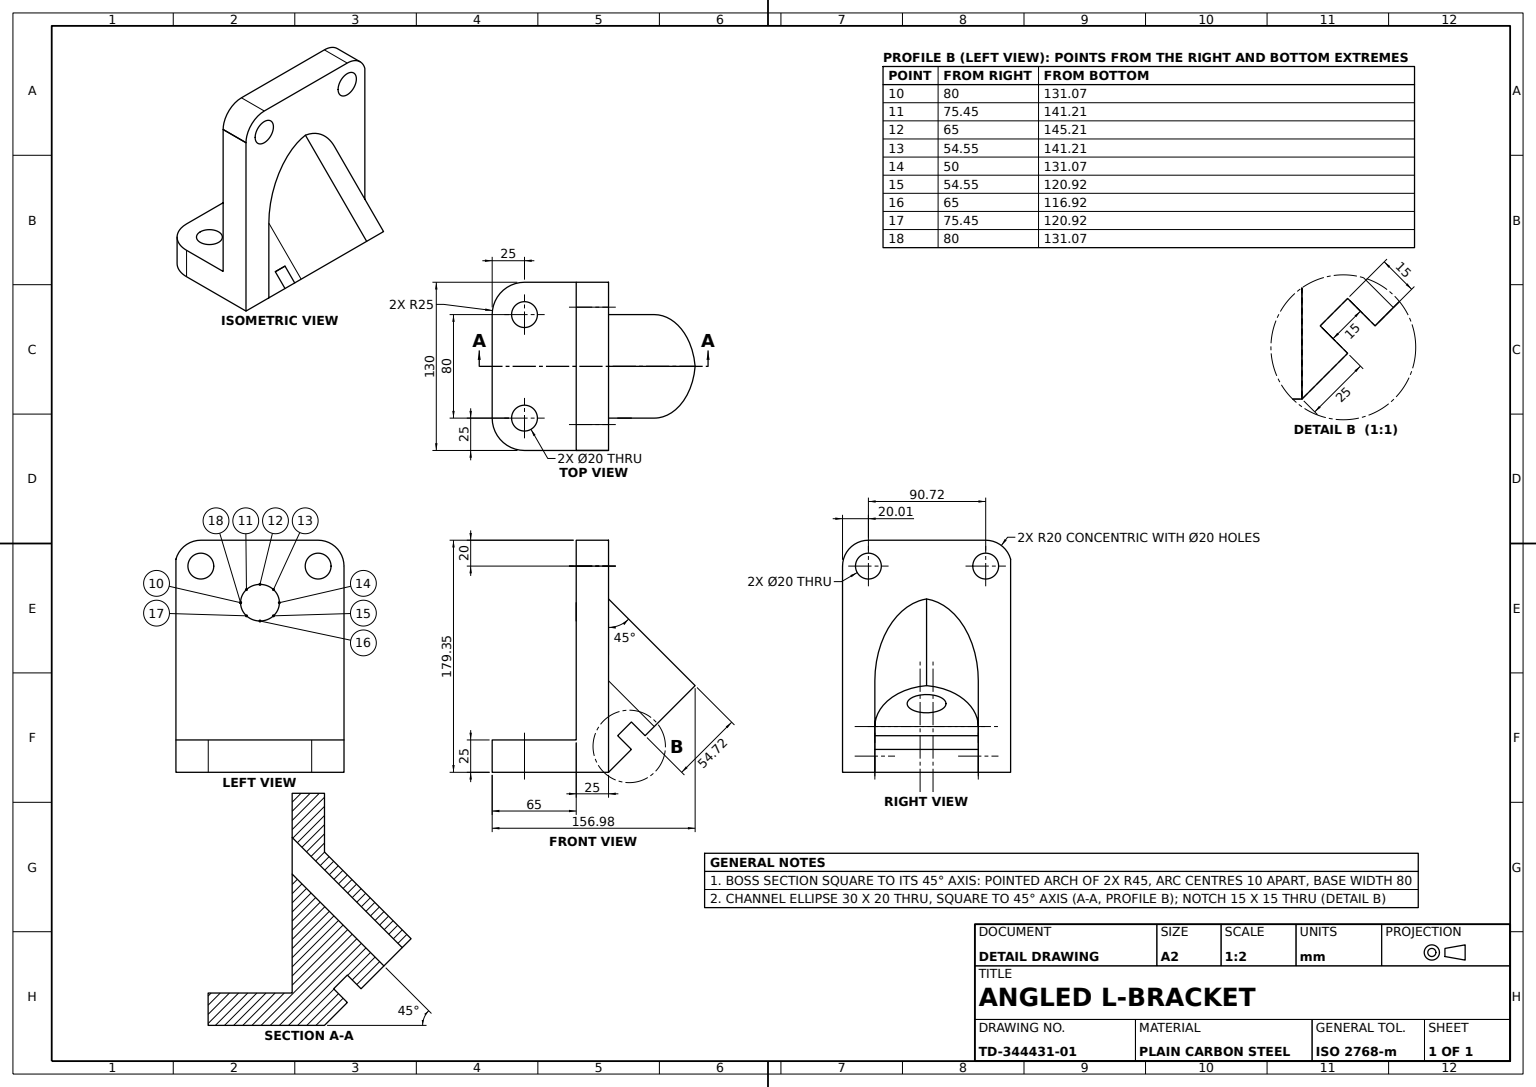
ISO-10303-21;
HEADER;
FILE_DESCRIPTION((''),'2;1');
FILE_NAME('','',(''),(''),'','','');
FILE_SCHEMA(('AUTOMOTIVE_DESIGN'));
ENDSEC;
DATA;
#1=APPLICATION_CONTEXT('');
#2=PRODUCT_CONTEXT('',#1,'mechanical');
#3=PRODUCT('','','',(#2));
#4=PRODUCT_DEFINITION_FORMATION('','',#3);
#5=PRODUCT_DEFINITION_CONTEXT('',#1,'design');
#6=PRODUCT_DEFINITION('','',#4,#5);
#7=PRODUCT_DEFINITION_SHAPE('','',#6);
#8=(LENGTH_UNIT()NAMED_UNIT(*)SI_UNIT(.MILLI.,.METRE.));
#9=(NAMED_UNIT(*)PLANE_ANGLE_UNIT()SI_UNIT($,.RADIAN.));
#10=(NAMED_UNIT(*)SI_UNIT($,.STERADIAN.)SOLID_ANGLE_UNIT());
#11=UNCERTAINTY_MEASURE_WITH_UNIT(LENGTH_MEASURE(1.E-05),#8,'distance_accuracy_value','');
#12=(GEOMETRIC_REPRESENTATION_CONTEXT(3)GLOBAL_UNCERTAINTY_ASSIGNED_CONTEXT((#11))GLOBAL_UNIT_ASSIGNED_CONTEXT((#8,#9,#10))REPRESENTATION_CONTEXT('',''));
#13=CARTESIAN_POINT('',(60.702747,0.,-23.512021));
#14=VERTEX_POINT('',#13);
#15=CARTESIAN_POINT('',(60.702747,25.,-23.512021));
#16=VERTEX_POINT('',#15);
#17=CARTESIAN_POINT('',(60.702747,-51.,-23.512021));
#18=DIRECTION('',(0.,1.,0.));
#19=VECTOR('',#18,1000.);
#20=LINE('',#17,#19);
#21=EDGE_CURVE('',#14,#16,#20,.T.);
#22=ORIENTED_EDGE('',*,*,#21,.F.);
#23=CARTESIAN_POINT('',(60.702747,0.,-43.512021));
#24=VERTEX_POINT('',#23);
#25=CARTESIAN_POINT('',(60.702747,0.,-33.512021));
#26=DIRECTION('',(0.,-1.,0.));
#27=DIRECTION('',(0.,0.,1.));
#28=AXIS2_PLACEMENT_3D('',#25,#26,#27);
#29=CIRCLE('',#28,10.);
#30=EDGE_CURVE('',#14,#24,#29,.T.);
#31=ORIENTED_EDGE('',*,*,#30,.T.);
#32=CARTESIAN_POINT('',(60.702747,25.,-43.512021));
#33=VERTEX_POINT('',#32);
#34=CARTESIAN_POINT('',(60.702747,-51.,-43.512021));
#35=LINE('',#34,#19);
#36=EDGE_CURVE('',#24,#33,#35,.T.);
#37=ORIENTED_EDGE('',*,*,#36,.T.);
#38=CARTESIAN_POINT('',(60.702747,25.,-33.512021));
#39=AXIS2_PLACEMENT_3D('',#38,#26,#27);
#40=CIRCLE('',#39,10.);
#41=EDGE_CURVE('',#16,#33,#40,.T.);
#42=ORIENTED_EDGE('',*,*,#41,.F.);
#43=EDGE_LOOP('',(#22,#31,#37,#42));
#44=FACE_OUTER_BOUND('',#43,.T.);
#45=CARTESIAN_POINT('',(60.702747,-51.,-33.512021));
#46=AXIS2_PLACEMENT_3D('',#45,#18,#27);
#47=CYLINDRICAL_SURFACE('',#46,10.);
#48=ADVANCED_FACE('',(#44),#47,.F.);
#49=CARTESIAN_POINT('',(85.702747,159.350288,-98.512021));
#50=VERTEX_POINT('',#49);
#51=CARTESIAN_POINT('',(85.702747,0.,-98.512021));
#52=VERTEX_POINT('',#51);
#53=CARTESIAN_POINT('',(85.702747,25.,-98.512021));
#54=VECTOR('',#26,1000.);
#55=LINE('',#53,#54);
#56=EDGE_CURVE('',#50,#52,#55,.T.);
#57=ORIENTED_EDGE('',*,*,#56,.F.);
#58=CARTESIAN_POINT('',(85.702747,159.350288,-73.512021));
#59=VERTEX_POINT('',#58);
#60=CARTESIAN_POINT('',(85.702747,159.350288,77.487979));
#61=DIRECTION('',(0.,0.,-1.));
#62=VECTOR('',#61,1000.);
#63=LINE('',#60,#62);
#64=EDGE_CURVE('',#59,#50,#63,.T.);
#65=ORIENTED_EDGE('',*,*,#64,.F.);
#66=CARTESIAN_POINT('',(85.702747,25.,-73.512021));
#67=VERTEX_POINT('',#66);
#68=CARTESIAN_POINT('',(85.702747,329.,-73.512021));
#69=LINE('',#68,#54);
#70=EDGE_CURVE('',#59,#67,#69,.T.);
#71=ORIENTED_EDGE('',*,*,#70,.T.);
#72=CARTESIAN_POINT('',(85.702747,25.,-33.512021));
#73=VERTEX_POINT('',#72);
#74=LINE('',#72,#62);
#75=EDGE_CURVE('',#73,#67,#74,.T.);
#76=ORIENTED_EDGE('',*,*,#75,.F.);
#77=CARTESIAN_POINT('',(85.702747,0.,-33.512021));
#78=VERTEX_POINT('',#77);
#79=LINE('',#72,#54);
#80=EDGE_CURVE('',#73,#78,#79,.T.);
#81=ORIENTED_EDGE('',*,*,#80,.T.);
#82=LINE('',#77,#62);
#83=EDGE_CURVE('',#78,#52,#82,.T.);
#84=ORIENTED_EDGE('',*,*,#83,.T.);
#85=EDGE_LOOP('',(#57,#65,#71,#76,#81,#84));
#86=FACE_OUTER_BOUND('',#85,.T.);
#87=DIRECTION('',(-1.,0.,0.));
#88=AXIS2_PLACEMENT_3D('',#72,#87,#27);
#89=PLANE('',#88);
#90=ADVANCED_FACE('',(#86),#89,.F.);
#91=CARTESIAN_POINT('',(-44.297253,164.722344,-98.512021));
#92=VERTEX_POINT('',#91);
#93=CARTESIAN_POINT('',(-44.297253,164.722344,-73.512021));
#94=VERTEX_POINT('',#93);
#95=CARTESIAN_POINT('',(-44.297253,164.722344,77.487979));
#96=VECTOR('',#27,1000.);
#97=LINE('',#95,#96);
#98=EDGE_CURVE('',#92,#94,#97,.T.);
#99=ORIENTED_EDGE('',*,*,#98,.T.);
#100=CARTESIAN_POINT('',(-25.032232,179.350288,-73.512021));
#101=VERTEX_POINT('',#100);
#102=CARTESIAN_POINT('',(-25.032232,159.350288,-73.512021));
#103=AXIS2_PLACEMENT_3D('',#102,#61,#87);
#104=CIRCLE('',#103,20.);
#105=EDGE_CURVE('',#94,#101,#104,.T.);
#106=ORIENTED_EDGE('',*,*,#105,.T.);
#107=CARTESIAN_POINT('',(-25.032232,179.350288,-98.512021));
#108=VERTEX_POINT('',#107);
#109=CARTESIAN_POINT('',(-25.032232,179.350288,77.487979));
#110=LINE('',#109,#62);
#111=EDGE_CURVE('',#101,#108,#110,.T.);
#112=ORIENTED_EDGE('',*,*,#111,.T.);
#113=CARTESIAN_POINT('',(-25.032232,159.350288,-98.512021));
#114=AXIS2_PLACEMENT_3D('',#113,#61,#87);
#115=CIRCLE('',#114,20.);
#116=EDGE_CURVE('',#92,#108,#115,.T.);
#117=ORIENTED_EDGE('',*,*,#116,.F.);
#118=EDGE_LOOP('',(#99,#106,#112,#117));
#119=FACE_OUTER_BOUND('',#118,.T.);
#120=CARTESIAN_POINT('',(-25.032232,159.350288,77.487979));
#121=AXIS2_PLACEMENT_3D('',#120,#61,#87);
#122=CYLINDRICAL_SURFACE('',#121,20.);
#123=ADVANCED_FACE('',(#119),#122,.T.);
#124=CARTESIAN_POINT('',(60.702747,25.,-8.512021));
#125=VERTEX_POINT('',#124);
#126=CARTESIAN_POINT('',(60.702747,0.,-8.512021));
#127=VERTEX_POINT('',#126);
#128=LINE('',#124,#54);
#129=EDGE_CURVE('',#125,#127,#128,.T.);
#130=ORIENTED_EDGE('',*,*,#129,.F.);
#131=CARTESIAN_POINT('',(-19.297253,25.,-8.512021));
#132=VERTEX_POINT('',#131);
#133=DIRECTION('',(1.,0.,0.));
#134=VECTOR('',#133,1000.);
#135=LINE('',#131,#134);
#136=EDGE_CURVE('',#132,#125,#135,.T.);
#137=ORIENTED_EDGE('',*,*,#136,.F.);
#138=CARTESIAN_POINT('',(-19.297253,0.,-8.512021));
#139=VERTEX_POINT('',#138);
#140=LINE('',#131,#54);
#141=EDGE_CURVE('',#132,#139,#140,.T.);
#142=ORIENTED_EDGE('',*,*,#141,.T.);
#143=LINE('',#138,#134);
#144=EDGE_CURVE('',#139,#127,#143,.T.);
#145=ORIENTED_EDGE('',*,*,#144,.T.);
#146=EDGE_LOOP('',(#130,#137,#142,#145));
#147=FACE_OUTER_BOUND('',#146,.T.);
#148=AXIS2_PLACEMENT_3D('',#131,#61,#87);
#149=PLANE('',#148);
#150=ADVANCED_FACE('',(#147),#149,.F.);
#151=ORIENTED_EDGE('',*,*,#141,.F.);
#152=CARTESIAN_POINT('',(-44.297253,25.,-33.512021));
#153=VERTEX_POINT('',#152);
#154=CARTESIAN_POINT('',(-19.297253,25.,-33.512021));
#155=AXIS2_PLACEMENT_3D('',#154,#18,#27);
#156=CIRCLE('',#155,25.);
#157=EDGE_CURVE('',#153,#132,#156,.T.);
#158=ORIENTED_EDGE('',*,*,#157,.F.);
#159=CARTESIAN_POINT('',(-44.297253,0.,-33.512021));
#160=VERTEX_POINT('',#159);
#161=LINE('',#152,#54);
#162=EDGE_CURVE('',#153,#160,#161,.T.);
#163=ORIENTED_EDGE('',*,*,#162,.T.);
#164=CARTESIAN_POINT('',(-19.297253,0.,-33.512021));
#165=AXIS2_PLACEMENT_3D('',#164,#18,#27);
#166=CIRCLE('',#165,25.);
#167=EDGE_CURVE('',#160,#139,#166,.T.);
#168=ORIENTED_EDGE('',*,*,#167,.T.);
#169=EDGE_LOOP('',(#151,#158,#163,#168));
#170=FACE_OUTER_BOUND('',#169,.T.);
#171=AXIS2_PLACEMENT_3D('',#154,#26,#61);
#172=CYLINDRICAL_SURFACE('',#171,25.);
#173=ADVANCED_FACE('',(#170),#172,.T.);
#174=CARTESIAN_POINT('',(60.702747,0.,-98.512021));
#175=VERTEX_POINT('',#174);
#176=CARTESIAN_POINT('',(60.702747,17.67767,-116.18969));
#177=VERTEX_POINT('',#176);
#178=DIRECTION('',(0.,0.707106781,-0.707106781));
#179=VECTOR('',#178,1000.);
#180=LINE('',#174,#179);
#181=EDGE_CURVE('',#175,#177,#180,.T.);
#182=ORIENTED_EDGE('',*,*,#181,.F.);
#183=CARTESIAN_POINT('',(-19.297253,0.,-98.512021));
#184=VERTEX_POINT('',#183);
#185=CARTESIAN_POINT('',(-44.297253,0.,-98.512021));
#186=VECTOR('',#87,1000.);
#187=LINE('',#185,#186);
#188=EDGE_CURVE('',#175,#184,#187,.T.);
#189=ORIENTED_EDGE('',*,*,#188,.T.);
#190=CARTESIAN_POINT('',(-19.297253,17.67767,-116.18969));
#191=VERTEX_POINT('',#190);
#192=LINE('',#183,#179);
#193=EDGE_CURVE('',#184,#191,#192,.T.);
#194=ORIENTED_EDGE('',*,*,#193,.T.);
#195=CARTESIAN_POINT('',(156.702747,17.67767,-116.18969));
#196=LINE('',#195,#186);
#197=EDGE_CURVE('',#177,#191,#196,.T.);
#198=ORIENTED_EDGE('',*,*,#197,.F.);
#199=EDGE_LOOP('',(#182,#189,#194,#198));
#200=FACE_OUTER_BOUND('',#199,.T.);
#201=DIRECTION('',(0.,-0.707106781,-0.707106781));
#202=AXIS2_PLACEMENT_3D('',#51,#201,#178);
#203=PLANE('',#202);
#204=ADVANCED_FACE('',(#200),#203,.T.);
#205=CARTESIAN_POINT('',(55.687973,159.350288,-73.512021));
#206=VERTEX_POINT('',#205);
#207=CARTESIAN_POINT('',(55.687973,159.350288,-98.512021));
#208=VERTEX_POINT('',#207);
#209=CARTESIAN_POINT('',(55.687973,159.350288,77.487979));
#210=LINE('',#209,#62);
#211=EDGE_CURVE('',#206,#208,#210,.T.);
#212=ORIENTED_EDGE('',*,*,#211,.T.);
#213=CARTESIAN_POINT('',(75.687973,159.350288,-98.512021));
#214=VERTEX_POINT('',#213);
#215=CARTESIAN_POINT('',(65.687973,159.350288,-98.512021));
#216=AXIS2_PLACEMENT_3D('',#215,#61,#87);
#217=CIRCLE('',#216,10.);
#218=EDGE_CURVE('',#208,#214,#217,.T.);
#219=ORIENTED_EDGE('',*,*,#218,.T.);
#220=CARTESIAN_POINT('',(75.687973,159.350288,-73.512021));
#221=VERTEX_POINT('',#220);
#222=CARTESIAN_POINT('',(75.687973,159.350288,77.487979));
#223=LINE('',#222,#62);
#224=EDGE_CURVE('',#221,#214,#223,.T.);
#225=ORIENTED_EDGE('',*,*,#224,.F.);
#226=CARTESIAN_POINT('',(65.687973,159.350288,-73.512021));
#227=AXIS2_PLACEMENT_3D('',#226,#61,#87);
#228=CIRCLE('',#227,10.);
#229=EDGE_CURVE('',#206,#221,#228,.T.);
#230=ORIENTED_EDGE('',*,*,#229,.F.);
#231=EDGE_LOOP('',(#212,#219,#225,#230));
#232=FACE_OUTER_BOUND('',#231,.T.);
#233=CARTESIAN_POINT('',(65.687973,159.350288,77.487979));
#234=AXIS2_PLACEMENT_3D('',#233,#61,#87);
#235=CYLINDRICAL_SURFACE('',#234,10.);
#236=ADVANCED_FACE('',(#232),#235,.F.);
#237=CARTESIAN_POINT('',(-19.297253,35.355339,-133.86736));
#238=VERTEX_POINT('',#237);
#239=CARTESIAN_POINT('',(20.702747,66.978116,-165.490137));
#240=VERTEX_POINT('',#239);
#241=CARTESIAN_POINT('',(25.702747,35.355339,-133.86736));
#242=AXIS2_PLACEMENT_3D('',#241,#201,#178);
#243=CIRCLE('',#242,45.);
#244=EDGE_CURVE('',#238,#240,#243,.T.);
#245=ORIENTED_EDGE('',*,*,#244,.F.);
#246=CARTESIAN_POINT('',(-19.297253,70.710678,-98.512021));
#247=VERTEX_POINT('',#246);
#248=CARTESIAN_POINT('',(-19.297253,172.61135,3.38865));
#249=VECTOR('',#201,1000.);
#250=LINE('',#248,#249);
#251=EDGE_CURVE('',#247,#238,#250,.T.);
#252=ORIENTED_EDGE('',*,*,#251,.F.);
#253=CARTESIAN_POINT('',(20.702747,133.956231,-98.512021));
#254=VERTEX_POINT('',#253);
#255=CARTESIAN_POINT('',(-3.237588,130.170932,-98.512021));
#256=CARTESIAN_POINT('',(-19.297253,104.778372,-98.512021));
#257=(BOUNDED_CURVE()B_SPLINE_CURVE(3,(#253,#255,#256,#246),.UNSPECIFIED.,.F.,.T.)B_SPLINE_CURVE_WITH_KNOTS((4,4),(0.111341014,1.570796327),.UNSPECIFIED.)CURVE()GEOMETRIC_REPRESENTATION_ITEM()RATIONAL_B_SPLINE_CURVE((1.,0.830237328,0.830237328,1.))REPRESENTATION_ITEM(''));
#258=EDGE_CURVE('',#254,#247,#257,.T.);
#259=ORIENTED_EDGE('',*,*,#258,.F.);
#260=CARTESIAN_POINT('',(20.702747,100.467173,-132.001079));
#261=DIRECTION('',(0.,0.707106781,0.707106781));
#262=VECTOR('',#261,1000.);
#263=LINE('',#260,#262);
#264=EDGE_CURVE('',#240,#254,#263,.T.);
#265=ORIENTED_EDGE('',*,*,#264,.F.);
#266=EDGE_LOOP('',(#245,#252,#259,#265));
#267=FACE_OUTER_BOUND('',#266,.T.);
#268=DIRECTION('',(0.,-0.707106781,0.707106781));
#269=AXIS2_PLACEMENT_3D('',#241,#261,#268);
#270=CYLINDRICAL_SURFACE('',#269,45.);
#271=ADVANCED_FACE('',(#267),#270,.T.);
#272=CARTESIAN_POINT('',(-19.297253,25.,-43.512021));
#273=VERTEX_POINT('',#272);
#274=CARTESIAN_POINT('',(-19.297253,25.,-23.512021));
#275=VERTEX_POINT('',#274);
#276=AXIS2_PLACEMENT_3D('',#154,#26,#27);
#277=CIRCLE('',#276,10.);
#278=EDGE_CURVE('',#273,#275,#277,.T.);
#279=ORIENTED_EDGE('',*,*,#278,.F.);
#280=CARTESIAN_POINT('',(-19.297253,0.,-43.512021));
#281=VERTEX_POINT('',#280);
#282=CARTESIAN_POINT('',(-19.297253,-122.,-43.512021));
#283=LINE('',#282,#19);
#284=EDGE_CURVE('',#281,#273,#283,.T.);
#285=ORIENTED_EDGE('',*,*,#284,.F.);
#286=CARTESIAN_POINT('',(-19.297253,0.,-23.512021));
#287=VERTEX_POINT('',#286);
#288=AXIS2_PLACEMENT_3D('',#164,#26,#27);
#289=CIRCLE('',#288,10.);
#290=EDGE_CURVE('',#281,#287,#289,.T.);
#291=ORIENTED_EDGE('',*,*,#290,.T.);
#292=CARTESIAN_POINT('',(-19.297253,-122.,-23.512021));
#293=LINE('',#292,#19);
#294=EDGE_CURVE('',#287,#275,#293,.T.);
#295=ORIENTED_EDGE('',*,*,#294,.T.);
#296=EDGE_LOOP('',(#279,#285,#291,#295));
#297=FACE_OUTER_BOUND('',#296,.T.);
#298=CARTESIAN_POINT('',(-19.297253,-122.,-33.512021));
#299=AXIS2_PLACEMENT_3D('',#298,#18,#27);
#300=CYLINDRICAL_SURFACE('',#299,10.);
#301=ADVANCED_FACE('',(#297),#300,.F.);
#302=CARTESIAN_POINT('',(35.702747,53.033009,-151.545029));
#303=VERTEX_POINT('',#302);
#304=CARTESIAN_POINT('',(5.702747,53.033009,-151.545029));
#305=VERTEX_POINT('',#304);
#306=CARTESIAN_POINT('',(35.702747,38.890873,-137.402894));
#307=CARTESIAN_POINT('',(5.702747,38.890873,-137.402894));
#308=(BOUNDED_CURVE()B_SPLINE_CURVE(3,(#302,#306,#307,#304),.UNSPECIFIED.,.F.,.T.)B_SPLINE_CURVE_WITH_KNOTS((4,4),(0.,3.141592654),.UNSPECIFIED.)CURVE()GEOMETRIC_REPRESENTATION_ITEM()RATIONAL_B_SPLINE_CURVE((1.,0.333333333,0.333333333,1.))REPRESENTATION_ITEM(''));
#309=EDGE_CURVE('',#303,#305,#308,.T.);
#310=ORIENTED_EDGE('',*,*,#309,.T.);
#311=CARTESIAN_POINT('',(5.702747,131.066017,-73.512021));
#312=VERTEX_POINT('',#311);
#313=CARTESIAN_POINT('',(5.702747,177.483802,-27.094236));
#314=LINE('',#313,#249);
#315=EDGE_CURVE('',#312,#305,#314,.T.);
#316=ORIENTED_EDGE('',*,*,#315,.F.);
#317=CARTESIAN_POINT('',(35.702747,131.066017,-73.512021));
#318=VERTEX_POINT('',#317);
#319=CARTESIAN_POINT('',(35.702747,130.10759,-73.512021));
#320=CARTESIAN_POINT('',(35.600479,129.166585,-73.512021));
#321=CARTESIAN_POINT('',(35.300783,127.78,-73.512021));
#322=CARTESIAN_POINT('',(35.176311,127.321991,-73.512021));
#323=CARTESIAN_POINT('',(34.87713,126.414533,-73.512021));
#324=CARTESIAN_POINT('',(34.703048,125.96758,-73.512021));
#325=CARTESIAN_POINT('',(34.310396,125.09694,-73.512021));
#326=CARTESIAN_POINT('',(34.090322,124.670065,-73.512021));
#327=CARTESIAN_POINT('',(33.609991,123.845556,-73.512021));
#328=CARTESIAN_POINT('',(33.350315,123.448422,-73.512021));
#329=CARTESIAN_POINT('',(32.515099,122.300572,-73.512021));
#330=CARTESIAN_POINT('',(31.882276,121.591535,-73.512021));
#331=CARTESIAN_POINT('',(30.825729,120.619653,-73.512021));
#332=CARTESIAN_POINT('',(30.458902,120.314032,-73.512021));
#333=CARTESIAN_POINT('',(29.696626,119.738626,-73.512021));
#334=CARTESIAN_POINT('',(29.300256,119.46836,-73.512021));
#335=CARTESIAN_POINT('',(28.079282,118.71807,-73.512021));
#336=CARTESIAN_POINT('',(27.216718,118.294713,-73.512021));
#337=CARTESIAN_POINT('',(25.87828,117.784604,-73.512021));
#338=CARTESIAN_POINT('',(25.423154,117.634773,-73.512021));
#339=CARTESIAN_POINT('',(24.502781,117.377738,-73.512021));
#340=CARTESIAN_POINT('',(24.039618,117.270986,-73.512021));
#341=CARTESIAN_POINT('',(22.64148,117.013951,-73.512021));
#342=CARTESIAN_POINT('',(21.697934,116.926332,-73.512021));
#343=CARTESIAN_POINT('',(20.265131,116.922731,-73.512021));
#344=CARTESIAN_POINT('',(19.786354,116.943124,-73.512021));
#345=CARTESIAN_POINT('',(18.835716,117.026641,-73.512021));
#346=CARTESIAN_POINT('',(18.362482,117.089745,-73.512021));
#347=CARTESIAN_POINT('',(16.949124,117.344001,-73.512021));
#348=CARTESIAN_POINT('',(16.02681,117.59787,-73.512021));
#349=CARTESIAN_POINT('',(14.684263,118.104187,-73.512021));
#350=CARTESIAN_POINT('',(14.245937,118.293029,-73.512021));
#351=CARTESIAN_POINT('',(13.387779,118.711099,-73.512021));
#352=CARTESIAN_POINT('',(12.966901,118.941015,-73.512021));
#353=CARTESIAN_POINT('',(12.15104,119.438301,-73.512021));
#354=CARTESIAN_POINT('',(11.755783,119.705646,-73.512021));
#355=CARTESIAN_POINT('',(10.99102,120.278336,-73.512021));
#356=CARTESIAN_POINT('',(10.621367,120.584009,-73.512021));
#357=CARTESIAN_POINT('',(9.563761,121.549429,-73.512021));
#358=CARTESIAN_POINT('',(8.920267,122.264073,-73.512021));
#359=CARTESIAN_POINT('',(8.074656,123.419514,-73.512021));
#360=CARTESIAN_POINT('',(7.811415,123.820283,-73.512021));
#361=CARTESIAN_POINT('',(7.328524,124.645228,-73.512021));
#362=CARTESIAN_POINT('',(7.108925,125.068978,-73.512021));
#363=CARTESIAN_POINT('',(6.714036,125.939353,-73.512021));
#364=CARTESIAN_POINT('',(6.538988,126.385903,-73.512021));
#365=CARTESIAN_POINT('',(6.23801,127.291853,-73.512021));
#366=CARTESIAN_POINT('',(6.111296,127.753303,-73.512021));
#367=CARTESIAN_POINT('',(5.907598,128.68837,-73.512021));
#368=CARTESIAN_POINT('',(5.831048,129.159568,-73.512021));
#369=CARTESIAN_POINT('',(5.72855,130.109294,-73.512021));
#370=CARTESIAN_POINT('',(5.702747,130.588587,-73.512021));
#371=B_SPLINE_CURVE_WITH_KNOTS('',3,(#317,#319,#320,#321,#322,#323,#324,#325,#326,#327,#328,#329,#330,#331,#332,#333,#334,#335,#336,#337,#338,#339,#340,#341,#342,#343,#344,#345,#346,#347,#348,#349,#350,#351,#352,#353,#354,#355,#356,#357,#358,#359,#360,#361,#362,#363,#364,#365,#366,#367,#368,#369,#370,#311),.UNSPECIFIED.,.F.,.F.,(4,2,2,2,2,2,2,2,2,2,2,2,2,2,2,2,2,2,2,2,2,2,2,2,2,2,4),(0.,0.002834445,0.004251667,0.00566889,0.007086112,0.008503334,0.011337779,0.012755002,0.014172224,0.017006669,0.018423891,0.019841114,0.022675559,0.024092781,0.025510003,0.028344448,0.029761671,0.031178893,0.032596115,0.034013338,0.036847783,0.038265005,0.039682228,0.04109945,0.042516672,0.043933895,0.045351117),.UNSPECIFIED.);
#372=EDGE_CURVE('',#318,#312,#371,.T.);
#373=ORIENTED_EDGE('',*,*,#372,.F.);
#374=CARTESIAN_POINT('',(35.702747,177.483802,-27.094236));
#375=LINE('',#374,#249);
#376=EDGE_CURVE('',#318,#303,#375,.T.);
#377=ORIENTED_EDGE('',*,*,#376,.T.);
#378=EDGE_LOOP('',(#310,#316,#373,#377));
#379=FACE_OUTER_BOUND('',#378,.T.);
#380=CARTESIAN_POINT('',(35.702747,131.534215,-73.043823));
#381=CARTESIAN_POINT('',(35.702747,117.39208,-58.901687));
#382=CARTESIAN_POINT('',(5.702747,117.39208,-58.901687));
#383=CARTESIAN_POINT('',(5.702747,131.534215,-73.043823));
#384=(BOUNDED_SURFACE()B_SPLINE_SURFACE(3,1,((#380,#302),(#381,#306),(#382,#307),(#383,#304)),.UNSPECIFIED.,.F.,.F.,.F.)B_SPLINE_SURFACE_WITH_KNOTS((4,4),(2,2),(0.,1.),(0.,1.),.UNSPECIFIED.)GEOMETRIC_REPRESENTATION_ITEM()RATIONAL_B_SPLINE_SURFACE(((1.,1.),(0.333333333,0.333333333),(0.333333333,0.333333333),(1.,1.)))REPRESENTATION_ITEM('')SURFACE());
#385=ADVANCED_FACE('',(#379),#384,.F.);
#386=EDGE_CURVE('',#287,#281,#289,.T.);
#387=ORIENTED_EDGE('',*,*,#386,.T.);
#388=ORIENTED_EDGE('',*,*,#284,.T.);
#389=EDGE_CURVE('',#275,#273,#277,.T.);
#390=ORIENTED_EDGE('',*,*,#389,.F.);
#391=ORIENTED_EDGE('',*,*,#294,.F.);
#392=EDGE_LOOP('',(#387,#388,#390,#391));
#393=FACE_OUTER_BOUND('',#392,.T.);
#394=ADVANCED_FACE('',(#393),#300,.F.);
#395=ORIENTED_EDGE('',*,*,#129,.T.);
#396=AXIS2_PLACEMENT_3D('',#25,#18,#27);
#397=CIRCLE('',#396,25.);
#398=EDGE_CURVE('',#127,#78,#397,.T.);
#399=ORIENTED_EDGE('',*,*,#398,.T.);
#400=ORIENTED_EDGE('',*,*,#80,.F.);
#401=AXIS2_PLACEMENT_3D('',#38,#18,#27);
#402=CIRCLE('',#401,25.);
#403=EDGE_CURVE('',#125,#73,#402,.T.);
#404=ORIENTED_EDGE('',*,*,#403,.F.);
#405=EDGE_LOOP('',(#395,#399,#400,#404));
#406=FACE_OUTER_BOUND('',#405,.T.);
#407=AXIS2_PLACEMENT_3D('',#38,#26,#61);
#408=CYLINDRICAL_SURFACE('',#407,25.);
#409=ADVANCED_FACE('',(#406),#408,.T.);
#410=ORIENTED_EDGE('',*,*,#41,.T.);
#411=EDGE_CURVE('',#33,#16,#40,.T.);
#412=ORIENTED_EDGE('',*,*,#411,.T.);
#413=EDGE_LOOP('',(#410,#412));
#414=FACE_BOUND('',#413,.T.);
#415=ORIENTED_EDGE('',*,*,#403,.T.);
#416=ORIENTED_EDGE('',*,*,#75,.T.);
#417=CARTESIAN_POINT('',(-44.297253,25.,-73.512021));
#418=VERTEX_POINT('',#417);
#419=LINE('',#417,#134);
#420=EDGE_CURVE('',#418,#67,#419,.T.);
#421=ORIENTED_EDGE('',*,*,#420,.F.);
#422=LINE('',#152,#96);
#423=EDGE_CURVE('',#418,#153,#422,.T.);
#424=ORIENTED_EDGE('',*,*,#423,.T.);
#425=ORIENTED_EDGE('',*,*,#157,.T.);
#426=ORIENTED_EDGE('',*,*,#136,.T.);
#427=EDGE_LOOP('',(#415,#416,#421,#424,#425,#426));
#428=FACE_OUTER_BOUND('',#427,.T.);
#429=ORIENTED_EDGE('',*,*,#278,.T.);
#430=ORIENTED_EDGE('',*,*,#389,.T.);
#431=EDGE_LOOP('',(#429,#430));
#432=FACE_BOUND('',#431,.T.);
#433=PLANE('',#155);
#434=ADVANCED_FACE('',(#414,#428,#432),#433,.T.);
#435=CARTESIAN_POINT('',(-15.032232,159.350288,-73.512021));
#436=VERTEX_POINT('',#435);
#437=CARTESIAN_POINT('',(-35.032232,159.350288,-73.512021));
#438=VERTEX_POINT('',#437);
#439=CIRCLE('',#103,10.);
#440=EDGE_CURVE('',#436,#438,#439,.T.);
#441=ORIENTED_EDGE('',*,*,#440,.F.);
#442=CARTESIAN_POINT('',(-15.032232,159.350288,-98.512021));
#443=VERTEX_POINT('',#442);
#444=CARTESIAN_POINT('',(-15.032232,159.350288,77.487979));
#445=LINE('',#444,#62);
#446=EDGE_CURVE('',#436,#443,#445,.T.);
#447=ORIENTED_EDGE('',*,*,#446,.T.);
#448=CARTESIAN_POINT('',(-35.032232,159.350288,-98.512021));
#449=VERTEX_POINT('',#448);
#450=CIRCLE('',#114,10.);
#451=EDGE_CURVE('',#443,#449,#450,.T.);
#452=ORIENTED_EDGE('',*,*,#451,.T.);
#453=CARTESIAN_POINT('',(-35.032232,159.350288,77.487979));
#454=LINE('',#453,#62);
#455=EDGE_CURVE('',#438,#449,#454,.T.);
#456=ORIENTED_EDGE('',*,*,#455,.F.);
#457=EDGE_LOOP('',(#441,#447,#452,#456));
#458=FACE_OUTER_BOUND('',#457,.T.);
#459=CYLINDRICAL_SURFACE('',#121,10.);
#460=ADVANCED_FACE('',(#458),#459,.F.);
#461=CARTESIAN_POINT('',(-19.297253,38.890873,-116.18969));
#462=VERTEX_POINT('',#461);
#463=CARTESIAN_POINT('',(-19.297253,28.284271,-105.583089));
#464=VERTEX_POINT('',#463);
#465=CARTESIAN_POINT('',(-19.297253,-38.649409,-38.649409));
#466=VECTOR('',#268,1000.);
#467=LINE('',#465,#466);
#468=EDGE_CURVE('',#462,#464,#467,.T.);
#469=ORIENTED_EDGE('',*,*,#468,.F.);
#470=CARTESIAN_POINT('',(60.702747,38.890873,-116.18969));
#471=VERTEX_POINT('',#470);
#472=CARTESIAN_POINT('',(156.702747,38.890873,-116.18969));
#473=LINE('',#472,#186);
#474=EDGE_CURVE('',#471,#462,#473,.T.);
#475=ORIENTED_EDGE('',*,*,#474,.F.);
#476=CARTESIAN_POINT('',(60.702747,28.284271,-105.583089));
#477=VERTEX_POINT('',#476);
#478=CARTESIAN_POINT('',(60.702747,49.350591,-126.649409));
#479=LINE('',#478,#466);
#480=EDGE_CURVE('',#471,#477,#479,.T.);
#481=ORIENTED_EDGE('',*,*,#480,.T.);
#482=CARTESIAN_POINT('',(156.702747,28.284271,-105.583089));
#483=LINE('',#482,#186);
#484=EDGE_CURVE('',#477,#464,#483,.T.);
#485=ORIENTED_EDGE('',*,*,#484,.T.);
#486=EDGE_LOOP('',(#469,#475,#481,#485));
#487=FACE_OUTER_BOUND('',#486,.T.);
#488=CARTESIAN_POINT('',(156.702747,-38.649409,-38.649409));
#489=AXIS2_PLACEMENT_3D('',#488,#201,#178);
#490=PLANE('',#489);
#491=ADVANCED_FACE('',(#487),#490,.T.);
#492=CARTESIAN_POINT('',(65.687973,179.350288,-98.512021));
#493=VERTEX_POINT('',#492);
#494=CARTESIAN_POINT('',(85.687973,159.350288,-98.512021));
#495=VERTEX_POINT('',#494);
#496=CIRCLE('',#216,20.);
#497=EDGE_CURVE('',#493,#495,#496,.T.);
#498=ORIENTED_EDGE('',*,*,#497,.F.);
#499=CARTESIAN_POINT('',(65.687973,179.350288,-73.512021));
#500=VERTEX_POINT('',#499);
#501=CARTESIAN_POINT('',(65.687973,179.350288,77.487979));
#502=LINE('',#501,#62);
#503=EDGE_CURVE('',#500,#493,#502,.T.);
#504=ORIENTED_EDGE('',*,*,#503,.F.);
#505=CARTESIAN_POINT('',(85.687973,159.350288,-73.512021));
#506=VERTEX_POINT('',#505);
#507=CIRCLE('',#227,20.);
#508=EDGE_CURVE('',#500,#506,#507,.T.);
#509=ORIENTED_EDGE('',*,*,#508,.T.);
#510=CARTESIAN_POINT('',(85.687973,159.350288,77.487979));
#511=LINE('',#510,#62);
#512=EDGE_CURVE('',#506,#495,#511,.T.);
#513=ORIENTED_EDGE('',*,*,#512,.T.);
#514=EDGE_LOOP('',(#498,#504,#509,#513));
#515=FACE_OUTER_BOUND('',#514,.T.);
#516=CYLINDRICAL_SURFACE('',#234,20.);
#517=ADVANCED_FACE('',(#515),#516,.T.);
#518=CARTESIAN_POINT('',(0.,159.350288,-98.512021));
#519=LINE('',#518,#134);
#520=EDGE_CURVE('',#495,#50,#519,.T.);
#521=ORIENTED_EDGE('',*,*,#520,.T.);
#522=ORIENTED_EDGE('',*,*,#56,.T.);
#523=EDGE_CURVE('',#52,#175,#187,.T.);
#524=ORIENTED_EDGE('',*,*,#523,.T.);
#525=CARTESIAN_POINT('',(60.702747,70.710678,-98.512021));
#526=VERTEX_POINT('',#525);
#527=CARTESIAN_POINT('',(60.702747,176.,-98.512021));
#528=LINE('',#527,#54);
#529=EDGE_CURVE('',#526,#175,#528,.T.);
#530=ORIENTED_EDGE('',*,*,#529,.F.);
#531=CARTESIAN_POINT('',(60.702747,104.778372,-98.512021));
#532=CARTESIAN_POINT('',(44.643082,130.170932,-98.512021));
#533=(BOUNDED_CURVE()B_SPLINE_CURVE(3,(#525,#531,#532,#253),.UNSPECIFIED.,.F.,.T.)B_SPLINE_CURVE_WITH_KNOTS((4,4),(1.570796327,3.030251639),.UNSPECIFIED.)CURVE()GEOMETRIC_REPRESENTATION_ITEM()RATIONAL_B_SPLINE_CURVE((1.,0.830237328,0.830237328,1.))REPRESENTATION_ITEM(''));
#534=EDGE_CURVE('',#526,#254,#533,.T.);
#535=ORIENTED_EDGE('',*,*,#534,.T.);
#536=ORIENTED_EDGE('',*,*,#258,.T.);
#537=CARTESIAN_POINT('',(-19.297253,176.,-98.512021));
#538=LINE('',#537,#54);
#539=EDGE_CURVE('',#247,#184,#538,.T.);
#540=ORIENTED_EDGE('',*,*,#539,.T.);
#541=VERTEX_POINT('',#185);
#542=CARTESIAN_POINT('',(0.,0.,-98.512021));
#543=LINE('',#542,#186);
#544=EDGE_CURVE('',#184,#541,#543,.T.);
#545=ORIENTED_EDGE('',*,*,#544,.T.);
#546=CARTESIAN_POINT('',(-44.297253,25.,-98.512021));
#547=LINE('',#546,#54);
#548=EDGE_CURVE('',#92,#541,#547,.T.);
#549=ORIENTED_EDGE('',*,*,#548,.F.);
#550=ORIENTED_EDGE('',*,*,#116,.T.);
#551=CARTESIAN_POINT('',(0.,179.350288,-98.512021));
#552=LINE('',#551,#134);
#553=EDGE_CURVE('',#108,#493,#552,.T.);
#554=ORIENTED_EDGE('',*,*,#553,.T.);
#555=ORIENTED_EDGE('',*,*,#497,.T.);
#556=EDGE_LOOP('',(#521,#522,#524,#530,#535,#536,#540,#545,#549,#550,#554,#555));
#557=FACE_OUTER_BOUND('',#556,.T.);
#558=EDGE_CURVE('',#449,#443,#450,.T.);
#559=ORIENTED_EDGE('',*,*,#558,.F.);
#560=ORIENTED_EDGE('',*,*,#451,.F.);
#561=EDGE_LOOP('',(#559,#560));
#562=FACE_BOUND('',#561,.T.);
#563=EDGE_CURVE('',#214,#208,#217,.T.);
#564=ORIENTED_EDGE('',*,*,#563,.F.);
#565=ORIENTED_EDGE('',*,*,#218,.F.);
#566=EDGE_LOOP('',(#564,#565));
#567=FACE_BOUND('',#566,.T.);
#568=AXIS2_PLACEMENT_3D('',#546,#27,#133);
#569=PLANE('',#568);
#570=ADVANCED_FACE('',(#557,#562,#567),#569,.F.);
#571=ORIENTED_EDGE('',*,*,#484,.F.);
#572=CARTESIAN_POINT('',(60.702747,154.93368,21.06632));
#573=LINE('',#572,#262);
#574=EDGE_CURVE('',#177,#477,#573,.T.);
#575=ORIENTED_EDGE('',*,*,#574,.F.);
#576=ORIENTED_EDGE('',*,*,#197,.T.);
#577=CARTESIAN_POINT('',(-19.297253,66.93368,-66.93368));
#578=LINE('',#577,#262);
#579=EDGE_CURVE('',#191,#464,#578,.T.);
#580=ORIENTED_EDGE('',*,*,#579,.T.);
#581=EDGE_LOOP('',(#571,#575,#576,#580));
#582=FACE_OUTER_BOUND('',#581,.T.);
#583=CARTESIAN_POINT('',(156.702747,66.93368,-66.93368));
#584=AXIS2_PLACEMENT_3D('',#583,#268,#201);
#585=PLANE('',#584);
#586=ADVANCED_FACE('',(#582),#585,.F.);
#587=ORIENTED_EDGE('',*,*,#21,.T.);
#588=ORIENTED_EDGE('',*,*,#411,.F.);
#589=ORIENTED_EDGE('',*,*,#36,.F.);
#590=EDGE_CURVE('',#24,#14,#29,.T.);
#591=ORIENTED_EDGE('',*,*,#590,.T.);
#592=EDGE_LOOP('',(#587,#588,#589,#591));
#593=FACE_OUTER_BOUND('',#592,.T.);
#594=ADVANCED_FACE('',(#593),#47,.F.);
#595=CARTESIAN_POINT('',(-44.297253,329.,-73.512021));
#596=LINE('',#595,#54);
#597=EDGE_CURVE('',#94,#418,#596,.T.);
#598=ORIENTED_EDGE('',*,*,#597,.F.);
#599=ORIENTED_EDGE('',*,*,#98,.F.);
#600=ORIENTED_EDGE('',*,*,#548,.T.);
#601=LINE('',#159,#96);
#602=EDGE_CURVE('',#541,#160,#601,.T.);
#603=ORIENTED_EDGE('',*,*,#602,.T.);
#604=ORIENTED_EDGE('',*,*,#162,.F.);
#605=ORIENTED_EDGE('',*,*,#423,.F.);
#606=EDGE_LOOP('',(#598,#599,#600,#603,#604,#605));
#607=FACE_OUTER_BOUND('',#606,.T.);
#608=AXIS2_PLACEMENT_3D('',#152,#133,#61);
#609=PLANE('',#608);
#610=ADVANCED_FACE('',(#607),#609,.F.);
#611=ORIENTED_EDGE('',*,*,#446,.F.);
#612=EDGE_CURVE('',#438,#436,#439,.T.);
#613=ORIENTED_EDGE('',*,*,#612,.F.);
#614=ORIENTED_EDGE('',*,*,#455,.T.);
#615=ORIENTED_EDGE('',*,*,#558,.T.);
#616=EDGE_LOOP('',(#611,#613,#614,#615));
#617=FACE_OUTER_BOUND('',#616,.T.);
#618=ADVANCED_FACE('',(#617),#459,.F.);
#619=ORIENTED_EDGE('',*,*,#264,.T.);
#620=ORIENTED_EDGE('',*,*,#534,.F.);
#621=CARTESIAN_POINT('',(60.702747,35.355339,-133.86736));
#622=VERTEX_POINT('',#621);
#623=CARTESIAN_POINT('',(60.702747,102.530483,-66.692216));
#624=LINE('',#623,#262);
#625=EDGE_CURVE('',#622,#526,#624,.T.);
#626=ORIENTED_EDGE('',*,*,#625,.F.);
#627=CARTESIAN_POINT('',(15.702747,35.355339,-133.86736));
#628=AXIS2_PLACEMENT_3D('',#627,#201,#178);
#629=CIRCLE('',#628,45.);
#630=EDGE_CURVE('',#240,#622,#629,.T.);
#631=ORIENTED_EDGE('',*,*,#630,.F.);
#632=EDGE_LOOP('',(#619,#620,#626,#631));
#633=FACE_OUTER_BOUND('',#632,.T.);
#634=CARTESIAN_POINT('',(15.702747,172.61135,3.38865));
#635=AXIS2_PLACEMENT_3D('',#634,#201,#178);
#636=CYLINDRICAL_SURFACE('',#635,45.);
#637=ADVANCED_FACE('',(#633),#636,.T.);
#638=ORIENTED_EDGE('',*,*,#315,.T.);
#639=CARTESIAN_POINT('',(5.702747,67.175144,-165.687165));
#640=CARTESIAN_POINT('',(35.702747,67.175144,-165.687165));
#641=(BOUNDED_CURVE()B_SPLINE_CURVE(3,(#304,#639,#640,#302),.UNSPECIFIED.,.F.,.T.)B_SPLINE_CURVE_WITH_KNOTS((4,4),(3.141592654,6.283185307),.UNSPECIFIED.)CURVE()GEOMETRIC_REPRESENTATION_ITEM()RATIONAL_B_SPLINE_CURVE((1.,0.333333333,0.333333333,1.))REPRESENTATION_ITEM(''));
#642=EDGE_CURVE('',#305,#303,#641,.T.);
#643=ORIENTED_EDGE('',*,*,#642,.T.);
#644=ORIENTED_EDGE('',*,*,#376,.F.);
#645=CARTESIAN_POINT('',(5.702747,132.020552,-73.512021));
#646=CARTESIAN_POINT('',(5.806017,132.97681,-73.512021));
#647=CARTESIAN_POINT('',(6.110639,134.375991,-73.512021));
#648=CARTESIAN_POINT('',(6.237574,134.838712,-73.512021));
#649=CARTESIAN_POINT('',(6.538531,135.744913,-73.512021));
#650=CARTESIAN_POINT('',(6.712629,136.18932,-73.512021));
#651=CARTESIAN_POINT('',(7.30539,137.496602,-73.512021));
#652=CARTESIAN_POINT('',(7.785651,138.314988,-73.512021));
#653=CARTESIAN_POINT('',(8.621601,139.461135,-73.512021));
#654=CARTESIAN_POINT('',(8.919855,139.829918,-73.512021));
#655=CARTESIAN_POINT('',(9.55591,140.540721,-73.512021));
#656=CARTESIAN_POINT('',(9.892998,140.881645,-73.512021));
#657=CARTESIAN_POINT('',(10.947776,141.848832,-73.512021));
#658=CARTESIAN_POINT('',(11.715739,142.42583,-73.512021));
#659=CARTESIAN_POINT('',(12.936719,143.173844,-73.512021));
#660=CARTESIAN_POINT('',(13.356875,143.404629,-73.512021));
#661=CARTESIAN_POINT('',(14.214143,143.824679,-73.512021));
#662=CARTESIAN_POINT('',(14.651972,144.014472,-73.512021));
#663=CARTESIAN_POINT('',(15.992834,144.523618,-73.512021));
#664=CARTESIAN_POINT('',(16.909089,144.777566,-73.512021));
#665=CARTESIAN_POINT('',(18.305349,145.033512,-73.512021));
#666=CARTESIAN_POINT('',(18.774992,145.09806,-73.512021));
#667=CARTESIAN_POINT('',(19.722832,145.185082,-73.512021));
#668=CARTESIAN_POINT('',(20.202003,145.207424,-73.512021));
#669=CARTESIAN_POINT('',(21.156082,145.208846,-73.512021));
#670=CARTESIAN_POINT('',(21.632454,145.188149,-73.512021));
#671=CARTESIAN_POINT('',(22.583858,145.103735,-73.512021));
#672=CARTESIAN_POINT('',(23.058457,145.039927,-73.512021));
#673=CARTESIAN_POINT('',(24.466169,144.78542,-73.512021));
#674=CARTESIAN_POINT('',(25.391918,144.529884,-73.512021));
#675=CARTESIAN_POINT('',(27.175902,143.855658,-73.512021));
#676=CARTESIAN_POINT('',(28.039388,143.434949,-73.512021));
#677=CARTESIAN_POINT('',(29.260633,142.689661,-73.512021));
#678=CARTESIAN_POINT('',(29.657373,142.421013,-73.512021));
#679=CARTESIAN_POINT('',(30.421402,141.848142,-73.512021));
#680=CARTESIAN_POINT('',(30.788732,141.544088,-73.512021));
#681=CARTESIAN_POINT('',(31.493548,140.900172,-73.512021));
#682=CARTESIAN_POINT('',(31.831205,140.559907,-73.512021));
#683=CARTESIAN_POINT('',(32.46866,139.850172,-73.512021));
#684=CARTESIAN_POINT('',(32.769441,139.479886,-73.512021));
#685=CARTESIAN_POINT('',(33.33418,138.707678,-73.512021));
#686=CARTESIAN_POINT('',(33.59619,138.308349,-73.512021));
#687=CARTESIAN_POINT('',(34.0779,137.485013,-73.512021));
#688=CARTESIAN_POINT('',(34.298362,137.059414,-73.512021));
#689=CARTESIAN_POINT('',(34.69269,136.189656,-73.512021));
#690=CARTESIAN_POINT('',(34.866715,135.745609,-73.512021));
#691=CARTESIAN_POINT('',(35.167864,134.838935,-73.512021));
#692=CARTESIAN_POINT('',(35.294619,134.37692,-73.512021));
#693=CARTESIAN_POINT('',(35.497779,133.444083,-73.512021));
#694=CARTESIAN_POINT('',(35.574675,132.970856,-73.512021));
#695=CARTESIAN_POINT('',(35.677044,132.0213,-73.512021));
#696=CARTESIAN_POINT('',(35.702747,131.545068,-73.512021));
#697=B_SPLINE_CURVE_WITH_KNOTS('',3,(#311,#645,#646,#647,#648,#649,#650,#651,#652,#653,#654,#655,#656,#657,#658,#659,#660,#661,#662,#663,#664,#665,#666,#667,#668,#669,#670,#671,#672,#673,#674,#675,#676,#677,#678,#679,#680,#681,#682,#683,#684,#685,#686,#687,#688,#689,#690,#691,#692,#693,#694,#695,#696,#317),.UNSPECIFIED.,.F.,.F.,(4,2,2,2,2,2,2,2,2,2,2,2,2,2,2,2,2,2,2,2,2,2,2,2,2,2,4),(0.045351117,0.048184597,0.049601336,0.051018076,0.053851556,0.055268295,0.056685035,0.059518515,0.060935254,0.062351994,0.065185474,0.066602213,0.068018953,0.069435693,0.070852433,0.073685912,0.076519391,0.077936131,0.079352871,0.080769611,0.08218635,0.08360309,0.08501983,0.08643657,0.087853309,0.089270049,0.090686789),.UNSPECIFIED.);
#698=EDGE_CURVE('',#312,#318,#697,.T.);
#699=ORIENTED_EDGE('',*,*,#698,.F.);
#700=EDGE_LOOP('',(#638,#643,#644,#699));
#701=FACE_OUTER_BOUND('',#700,.T.);
#702=CARTESIAN_POINT('',(5.702747,138.6597,-65.918338));
#703=CARTESIAN_POINT('',(5.702747,152.801836,-80.060473));
#704=CARTESIAN_POINT('',(35.702747,152.801836,-80.060473));
#705=CARTESIAN_POINT('',(35.702747,138.6597,-65.918338));
#706=(BOUNDED_SURFACE()B_SPLINE_SURFACE(3,1,((#702,#304),(#703,#639),(#704,#640),(#705,#302)),.UNSPECIFIED.,.F.,.F.,.F.)B_SPLINE_SURFACE_WITH_KNOTS((4,4),(2,2),(0.,1.),(0.,1.),.UNSPECIFIED.)GEOMETRIC_REPRESENTATION_ITEM()RATIONAL_B_SPLINE_SURFACE(((1.,1.),(0.333333333,0.333333333),(0.333333333,0.333333333),(1.,1.)))REPRESENTATION_ITEM('')SURFACE());
#707=ADVANCED_FACE('',(#701),#706,.F.);
#708=ORIENTED_EDGE('',*,*,#512,.F.);
#709=CARTESIAN_POINT('',(-44.297253,159.350288,-73.512021));
#710=LINE('',#709,#134);
#711=EDGE_CURVE('',#506,#59,#710,.T.);
#712=ORIENTED_EDGE('',*,*,#711,.T.);
#713=ORIENTED_EDGE('',*,*,#64,.T.);
#714=ORIENTED_EDGE('',*,*,#520,.F.);
#715=EDGE_LOOP('',(#708,#712,#713,#714));
#716=FACE_OUTER_BOUND('',#715,.T.);
#717=CARTESIAN_POINT('',(0.,159.350288,77.487979));
#718=AXIS2_PLACEMENT_3D('',#717,#18,#27);
#719=PLANE('',#718);
#720=ADVANCED_FACE('',(#716),#719,.T.);
#721=ORIENTED_EDGE('',*,*,#642,.F.);
#722=ORIENTED_EDGE('',*,*,#309,.F.);
#723=EDGE_LOOP('',(#721,#722));
#724=FACE_BOUND('',#723,.T.);
#725=CARTESIAN_POINT('',(60.702747,28.284271,-126.796292));
#726=VERTEX_POINT('',#725);
#727=CARTESIAN_POINT('',(-19.297253,28.284271,-126.796292));
#728=VERTEX_POINT('',#727);
#729=CARTESIAN_POINT('',(156.702747,28.284271,-126.796292));
#730=LINE('',#729,#186);
#731=EDGE_CURVE('',#726,#728,#730,.T.);
#732=ORIENTED_EDGE('',*,*,#731,.T.);
#733=EDGE_CURVE('',#728,#238,#192,.T.);
#734=ORIENTED_EDGE('',*,*,#733,.T.);
#735=ORIENTED_EDGE('',*,*,#244,.T.);
#736=ORIENTED_EDGE('',*,*,#630,.T.);
#737=EDGE_CURVE('',#726,#622,#180,.T.);
#738=ORIENTED_EDGE('',*,*,#737,.F.);
#739=EDGE_LOOP('',(#732,#734,#735,#736,#738));
#740=FACE_OUTER_BOUND('',#739,.T.);
#741=ADVANCED_FACE('',(#724,#740),#203,.T.);
#742=EDGE_CURVE('',#221,#206,#228,.T.);
#743=ORIENTED_EDGE('',*,*,#742,.F.);
#744=ORIENTED_EDGE('',*,*,#224,.T.);
#745=ORIENTED_EDGE('',*,*,#563,.T.);
#746=ORIENTED_EDGE('',*,*,#211,.F.);
#747=EDGE_LOOP('',(#743,#744,#745,#746));
#748=FACE_OUTER_BOUND('',#747,.T.);
#749=ADVANCED_FACE('',(#748),#235,.F.);
#750=CARTESIAN_POINT('',(-44.297253,179.350288,-73.512021));
#751=LINE('',#750,#134);
#752=EDGE_CURVE('',#101,#500,#751,.T.);
#753=ORIENTED_EDGE('',*,*,#752,.T.);
#754=ORIENTED_EDGE('',*,*,#503,.T.);
#755=ORIENTED_EDGE('',*,*,#553,.F.);
#756=ORIENTED_EDGE('',*,*,#111,.F.);
#757=EDGE_LOOP('',(#753,#754,#755,#756));
#758=FACE_OUTER_BOUND('',#757,.T.);
#759=CARTESIAN_POINT('',(0.,179.350288,77.487979));
#760=AXIS2_PLACEMENT_3D('',#759,#18,#27);
#761=PLANE('',#760);
#762=ADVANCED_FACE('',(#758),#761,.T.);
#763=ORIENTED_EDGE('',*,*,#144,.F.);
#764=ORIENTED_EDGE('',*,*,#167,.F.);
#765=ORIENTED_EDGE('',*,*,#602,.F.);
#766=ORIENTED_EDGE('',*,*,#544,.F.);
#767=ORIENTED_EDGE('',*,*,#188,.F.);
#768=ORIENTED_EDGE('',*,*,#523,.F.);
#769=ORIENTED_EDGE('',*,*,#83,.F.);
#770=ORIENTED_EDGE('',*,*,#398,.F.);
#771=EDGE_LOOP('',(#763,#764,#765,#766,#767,#768,#769,#770));
#772=FACE_OUTER_BOUND('',#771,.T.);
#773=ORIENTED_EDGE('',*,*,#30,.F.);
#774=ORIENTED_EDGE('',*,*,#590,.F.);
#775=EDGE_LOOP('',(#773,#774));
#776=FACE_BOUND('',#775,.T.);
#777=ORIENTED_EDGE('',*,*,#290,.F.);
#778=ORIENTED_EDGE('',*,*,#386,.F.);
#779=EDGE_LOOP('',(#777,#778));
#780=FACE_BOUND('',#779,.T.);
#781=PLANE('',#165);
#782=ADVANCED_FACE('',(#772,#776,#780),#781,.F.);
#783=ORIENTED_EDGE('',*,*,#737,.T.);
#784=ORIENTED_EDGE('',*,*,#625,.T.);
#785=ORIENTED_EDGE('',*,*,#529,.T.);
#786=ORIENTED_EDGE('',*,*,#181,.T.);
#787=ORIENTED_EDGE('',*,*,#574,.T.);
#788=ORIENTED_EDGE('',*,*,#480,.F.);
#789=CARTESIAN_POINT('',(60.702747,165.540282,10.459718));
#790=LINE('',#789,#262);
#791=EDGE_CURVE('',#726,#471,#790,.T.);
#792=ORIENTED_EDGE('',*,*,#791,.F.);
#793=EDGE_LOOP('',(#783,#784,#785,#786,#787,#788,#792));
#794=FACE_OUTER_BOUND('',#793,.T.);
#795=CARTESIAN_POINT('',(60.702747,176.,0.));
#796=AXIS2_PLACEMENT_3D('',#795,#87,#27);
#797=PLANE('',#796);
#798=ADVANCED_FACE('',(#794),#797,.F.);
#799=ORIENTED_EDGE('',*,*,#474,.T.);
#800=CARTESIAN_POINT('',(-19.297253,77.540282,-77.540282));
#801=LINE('',#800,#262);
#802=EDGE_CURVE('',#728,#462,#801,.T.);
#803=ORIENTED_EDGE('',*,*,#802,.F.);
#804=ORIENTED_EDGE('',*,*,#731,.F.);
#805=ORIENTED_EDGE('',*,*,#791,.T.);
#806=EDGE_LOOP('',(#799,#803,#804,#805));
#807=FACE_OUTER_BOUND('',#806,.T.);
#808=CARTESIAN_POINT('',(156.702747,77.540282,-77.540282));
#809=AXIS2_PLACEMENT_3D('',#808,#268,#201);
#810=PLANE('',#809);
#811=ADVANCED_FACE('',(#807),#810,.T.);
#812=ORIENTED_EDGE('',*,*,#742,.T.);
#813=ORIENTED_EDGE('',*,*,#229,.T.);
#814=EDGE_LOOP('',(#812,#813));
#815=FACE_BOUND('',#814,.T.);
#816=ORIENTED_EDGE('',*,*,#440,.T.);
#817=ORIENTED_EDGE('',*,*,#612,.T.);
#818=EDGE_LOOP('',(#816,#817));
#819=FACE_BOUND('',#818,.T.);
#820=ORIENTED_EDGE('',*,*,#698,.T.);
#821=ORIENTED_EDGE('',*,*,#372,.T.);
#822=EDGE_LOOP('',(#820,#821));
#823=FACE_BOUND('',#822,.T.);
#824=ORIENTED_EDGE('',*,*,#420,.T.);
#825=ORIENTED_EDGE('',*,*,#70,.F.);
#826=ORIENTED_EDGE('',*,*,#711,.F.);
#827=ORIENTED_EDGE('',*,*,#508,.F.);
#828=ORIENTED_EDGE('',*,*,#752,.F.);
#829=ORIENTED_EDGE('',*,*,#105,.F.);
#830=ORIENTED_EDGE('',*,*,#597,.T.);
#831=EDGE_LOOP('',(#824,#825,#826,#827,#828,#829,#830));
#832=FACE_OUTER_BOUND('',#831,.T.);
#833=AXIS2_PLACEMENT_3D('',#595,#61,#87);
#834=PLANE('',#833);
#835=ADVANCED_FACE('',(#815,#819,#823,#832),#834,.F.);
#836=ORIENTED_EDGE('',*,*,#539,.F.);
#837=ORIENTED_EDGE('',*,*,#251,.T.);
#838=ORIENTED_EDGE('',*,*,#733,.F.);
#839=ORIENTED_EDGE('',*,*,#802,.T.);
#840=ORIENTED_EDGE('',*,*,#468,.T.);
#841=ORIENTED_EDGE('',*,*,#579,.F.);
#842=ORIENTED_EDGE('',*,*,#193,.F.);
#843=EDGE_LOOP('',(#836,#837,#838,#839,#840,#841,#842));
#844=FACE_OUTER_BOUND('',#843,.T.);
#845=CARTESIAN_POINT('',(-19.297253,176.,0.));
#846=AXIS2_PLACEMENT_3D('',#845,#87,#27);
#847=PLANE('',#846);
#848=ADVANCED_FACE('',(#844),#847,.T.);
#849=CLOSED_SHELL('',(#48,#90,#123,#150,#173,#204,#236,#271,#301,#385,#394,#409,#434,#460,#491,#517,#570,#586,#594,#610,#618,#637,#707,#720,#741,#749,#762,#782,#798,#811,#835,#848));
#850=MANIFOLD_SOLID_BREP('',#849);
#851=ADVANCED_BREP_SHAPE_REPRESENTATION('',(#850),#12);
#852=SHAPE_DEFINITION_REPRESENTATION(#7,#851);
ENDSEC;
END-ISO-10303-21;
